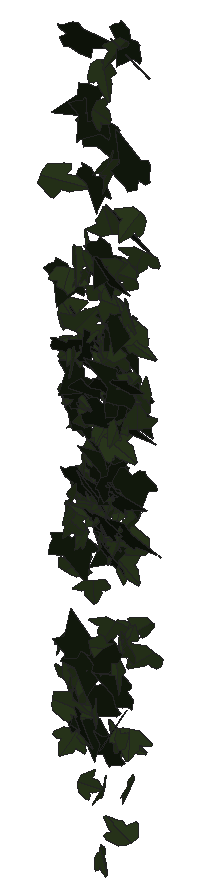
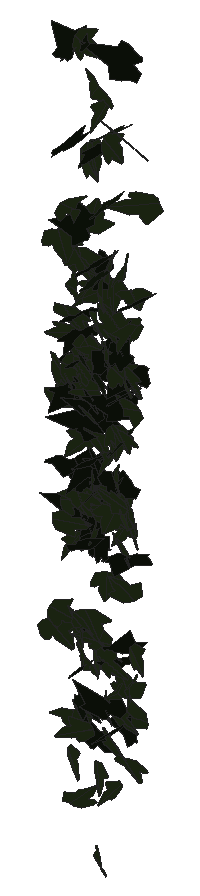
# SketchUp Ruby script. Lengths in inches.
U = 1.inch
M = Sketchup.active_model
def pt(a) = Geom::Point3d.new(a.map { |v| v * U })
def face(e, loops, mat)
  f = e.add_face(loops[0].map { |a| pt(a) })
  loops[1..].each { |l| e.add_face(l.map { |a| pt(a) }).erase! }
  f.material = f.back_material = mat if mat
  f
end
# faces: each face lists its corners as indices into pts; further lists are holes
def faces(e, pts, list, mat = nil) = list.each { |f| face(e, (f[0].is_a?(Array) ? f : [f]).map { |l| l.map { |i| pts[i] } }, mat) }
# xy, xz, yz: faces in a plane at the given z, y or x. An outline is a flat list of corners, or four numbers for a rectangle; further outlines are holes
def ring(l) = l.size == 4 ? [[l[0], l[1]], [l[2], l[1]], [l[2], l[3]], [l[0], l[3]]] : l.each_slice(2).to_a
def flat(e, list, mat, &to3) = list.each { |f| face(e, (f[0].is_a?(Array) ? f : [f]).map { |l| ring(l).map { |u, v| to3.(u, v) } }, mat) }
def xy(e, z, list, mat = nil) = flat(e, list, mat) { |x, y| [x, y, z] }
def xz(e, y, list, mat = nil) = flat(e, list, mat) { |x, z| [x, y, z] }
def yz(e, x, list, mat = nil) = flat(e, list, mat) { |y, z| [x, y, z] }
def lines(e, pts, list) = list.each { |a, b| e.add_line(pt(pts[a]), pt(pts[b])) }
# prism: a flat outline (further loops are holes) pulled along v
def prism(e, loops, v, mat = nil)
  f = face(e, loops, mat); d = Geom::Vector3d.new(v.map { |x| x * U })
  f.pushpull(f.normal.samedirection?(d) ? d.length : -d.length)
end
def box(e, o, s, mat = nil) = prism(e, [[o, [o[0] + s[0], o[1], o[2]], [o[0] + s[0], o[1] + s[1], o[2]], [o[0], o[1] + s[1], o[2]]]], [0, 0, s[2]], mat)
def at(x, y, z, deg = 0) = Geom::Transformation.translation(pt([x, y, z])) * Geom::Transformation.rotation(ORIGIN, Z_AXIS, deg.degrees)
def axes(o, x, y, z) = Geom::Transformation.new([*x, 0, *y, 0, *z, 0, *pt(o).to_a, 1])
def part(name) = M.definitions.add(name)
# library, detail: a bought-in or finely detailed component or shape, given as its bounding box
def library(name, o, s) = part(name).tap { |d| box(d.entities, o, s) }
def detail(e, o, s) = box(e.add_group.entities, o, s)
def put(e, d, t, mat = nil) = e.add_instance(d, t).tap { |i| i.material = mat if mat }
def group(e, t, mat = nil) = e.add_group.tap { |g| g.transformation = t; g.material = mat if mat }.entities
root = M.entities
M.materials.add("1026 AP 7946 SUNNY SIDE UP").color = [254, 231, 186]
M.materials.add("efeu1").color = [18, 25, 13]
M.materials.add("efeu2").color = [43, 57, 29]
c1 = part("ivyleaf_10")
p = [[0,0.5,-0.03],[-0.0625,2.02,-0.43],[-0.19,2.01,-0.46],[-0.54,1.05,-0.29],[-0.52,0.625,-0.18],[-0.83,0.76,-0.28],
  [-1.16,0.64,-0.33],[-1.15,0.33,-0.24],[-0.77,-0.39,0.02],[-0.3,-0.51,0.16],[0.04,-0.48,0.23],[-0.02,2.01,-0.4375],
  [-0.06,2.01,-0.43],[0.04,-0.49,0.23],[0.67,-0.49,0.14],[1.38,0.36,-0.2],[1.375,0.51,-0.24],[0.81,0.65,-0.19],
  [0.62,0.59,-0.15],[0.6,1.09,-0.28],[0.5,1.23,-0.31]]
faces(c1.entities,p,[[0,1,2,3,4,5,6,7,8,9,10],[11,12,0,13,14,15,16,17,18,19,20]],"efeu2")
c2 = part("ivyleaf_9")
p = [[1.54,2.16,1.25],[1.36,2.04,1.19],[-0.21,0.99,0.68],[-0.71,1.11,0.82],[-0.85,0.86,0.67],[-0.8,0.17,0.21],
  [-0.9,-0.01,0.1],[-0.67,-0.16,-0.02],[-0.08,-0.08,-0.05],[-0.03,-0.6,-0.4],[0.65,-0.88,-0.66],[0.83,-0.6,-0.49],
  [1.29,-0.42,-0.43],[1.8125,-0.07,-0.26],[1.21,0.44,0.15]]
faces(c2.entities,p,[[0,1,2,3,4,5,6,7,8,9,10,11,12,13,14]],"efeu1")
put(root,c1,axes([109.62,211.6875,250.39],[0.16374,0.16679,0.12106],[-0.11164,-0.09293,0.20178],[0.29985,-0.12568,0.00902]),"1026 AP 7946 SUNNY SIDE UP")
put(root,c1,axes([108.4,211.74,262.72],[-0.02673,0.24163,-0.15836],[0.017,-0.15471,-0.25045],[-0.45115,-0.02015,-0.00005]),"1026 AP 7946 SUNNY SIDE UP")
put(root,c1,axes([109.34,211.75,256.78],[0.22873,-0.17421,0.08508],[0.06387,-0.07471,-0.23369],[0.29704,0.15022,-0.01527]),"1026 AP 7946 SUNNY SIDE UP")
put(root,c1,axes([108.19,211.72,262.21],[0.27131,0.14604,-0.06363],[-0.05264,-0.05692,-0.2322],[-0.24423,0.1745,-0.02064]),"1026 AP 7946 SUNNY SIDE UP")
put(root,c2,axes([108.61,211.79,257.76],[0.18016,-0.19995,0.08422],[0.04769,-0.07802,-0.23756],[0.33698,0.11794,-0.01141]),"1026 AP 7946 SUNNY SIDE UP")
put(root,c2,axes([108.22,211.78,252.6],[0.01435,-0.02257,-0.25967],[0.39632,-0.02035,0.01116],[-0.03338,-0.25127,0.02093]),"1026 AP 7946 SUNNY SIDE UP")
put(root,c1,axes([108.43,211.59,256.9],[-0.07924,-0.16549,-0.16152],[0.11826,0.1385,-0.17576],[0.33731,-0.08744,0.02368]),"1026 AP 7946 SUNNY SIDE UP")
put(root,c1,axes([109.19,211.67,265.08],[0.00366,-0.24784,-0.05925],[-0.00514,0.05607,-0.25499],[0.39953,0.00299,-0.00274]),"1026 AP 7946 SUNNY SIDE UP")
put(root,c1,axes([109.53,211.81,261.86],[0.08841,-0.06805,0.22834],[0.297,-0.11951,-0.0877],[0.21244,0.19539,0.02759]),"1026 AP 7946 SUNNY SIDE UP")
put(root,c1,axes([108.54,211.67,261.21],[-0.30265,-0.17856,0.11997],[0.11357,0.09444,0.27036],[-0.3163,0.20476,-0.01772]),"1026 AP 7946 SUNNY SIDE UP")
put(root,c2,axes([109.25,211.76,256.22],[0.21365,-0.1787,0.10515],[-0.07433,0.09318,0.23115],[-0.31576,-0.14285,0.01674]),"1026 AP 7946 SUNNY SIDE UP")
put(root,c2,axes([109.39,211.76,256.98],[0.22623,-0.10183,0.19765],[0.23969,-0.11757,-0.18219],[0.24443,0.20954,-0.00427]),"1026 AP 7946 SUNNY SIDE UP")
put(root,c1,axes([108.05,211.68,252.77],[0.01944,0.0241,0.24923],[0.36524,0.06991,-0.019],[-0.11218,0.23179,-0.01869]),"1026 AP 7946 SUNNY SIDE UP")
put(root,c2,axes([109.15,211.77,257.65],[0.1143,-0.06217,0.22835],[0.2682,-0.14212,-0.09936],[0.2439,0.18541,0.00225]),"1026 AP 7946 SUNNY SIDE UP")
put(root,c2,axes([108.92,211.65,257.16],[0.40597,-0.0286,-0.07113],[-0.11167,-0.01843,-0.26645],[0.03583,0.26658,-0.02447]),"1026 AP 7946 SUNNY SIDE UP")
put(root,c2,axes([109.58,211.83,260.13],[-0.13347,-0.27317,-0.03518],[-0.02589,-0.02901,0.29443],[-0.43181,0.08617,-0.00678]),"1026 AP 7946 SUNNY SIDE UP")
put(root,c1,axes([108.83,211.71,255.64],[-0.22701,-0.16897,-0.01737],[0.03319,0.00284,-0.22848],[0.26479,-0.14522,0.01374]),"1026 AP 7946 SUNNY SIDE UP")
put(root,c1,axes([109.25,211.82,264.9375],[0.07697,-0.27103,0.09657],[0.03725,-0.09252,-0.2842],[0.4502,0.05399,0.007]),"1026 AP 7946 SUNNY SIDE UP")
put(root,c2,axes([108.625,211.84,253.9],[-0.16438,-0.22602,-0.02982],[0.03648,0.01971,-0.2561],[0.35618,-0.10633,0.01247]),"1026 AP 7946 SUNNY SIDE UP")
put(root,c2,axes([108.33,211.78,257.66],[0.12623,-0.04783,0.24696],[0.29425,-0.15076,-0.09632],[0.24796,0.20326,-0.01142]),"1026 AP 7946 SUNNY SIDE UP")
put(root,c2,axes([109.29,211.62,260.24],[0.32636,0.14489,-0.05329],[-0.05073,-0.04535,-0.26035],[-0.23698,0.20925,-0.01766]),"1026 AP 7946 SUNNY SIDE UP")
put(root,c2,axes([108.0625,211.91,262.08],[-0.12606,-0.22075,0.10012],[-0.02119,-0.09947,-0.24168],[0.37946,-0.07889,0.01977]),"1026 AP 7946 SUNNY SIDE UP")
put(root,c1,axes([108.14,211.78,259.65],[-0.16249,0.00322,-0.21366],[0.2904,-0.10409,-0.09707],[-0.14854,-0.20704,0.04396]),"1026 AP 7946 SUNNY SIDE UP")
put(root,c1,axes([108.24,211.75,253.33],[-0.30544,-0.02384,0.1197],[0.18237,0.00979,0.20164],[-0.04008,0.22621,0.00523]),"1026 AP 7946 SUNNY SIDE UP")
put(root,c2,axes([108.52,211.6875,254.12],[-0.27032,-0.12765,0.11551],[0.14375,0.06617,0.22097],[-0.22607,0.19471,0.00239]),"1026 AP 7946 SUNNY SIDE UP")
put(root,c1,axes([108.29,211.7,257.0625],[0.17219,-0.1863,-0.09583],[-0.07606,0.07824,-0.22216],[0.31771,0.1197,-0.00125]),"1026 AP 7946 SUNNY SIDE UP")
put(root,c2,axes([109.41,211.82,252.84],[-0.1908,0.11557,-0.18423],[0.18209,-0.13781,-0.17287],[-0.28199,-0.16718,0.01303]),"1026 AP 7946 SUNNY SIDE UP")
put(root,c2,axes([109.27,211.63,254.12],[-0.13737,0.14339,0.17972],[-0.19285,0.1259,-0.16994],[-0.29697,-0.14809,0.02722]),"1026 AP 7946 SUNNY SIDE UP")
put(root,c1,axes([109.08,211.66,251.29],[0.03072,-0.20439,-0.13522],[-0.03077,0.12876,-0.21067],[0.37972,0.02697,-0.00613]),"1026 AP 7946 SUNNY SIDE UP")
put(root,c1,axes([108.08,211.8,254.25],[0.05919,-0.22176,0.04165],[0.00514,-0.04172,-0.23194],[0.35476,0.0376,-0.00359]),"1026 AP 7946 SUNNY SIDE UP")
put(root,c1,axes([109.29,211.64,257.74],[0.10448,-0.14943,-0.1821],[-0.07442,0.17034,-0.16649],[0.35522,0.07964,0.01868]),"1026 AP 7946 SUNNY SIDE UP")
put(root,c1,axes([109.13,211.89,257.33],[-0.01417,-0.14259,0.17478],[-0.02048,-0.16998,-0.14817],[0.34885,-0.01577,-0.0016]),"1026 AP 7946 SUNNY SIDE UP")
put(root,c1,axes([107.85,211.63,264.27],[-0.07843,-0.0737,-0.29054],[0.40455,0.12249,-0.07925],[0.21411,-0.25843,0.04332]),"1026 AP 7946 SUNNY SIDE UP")
put(root,c1,axes([108.875,211.85,257.125],[-0.07152,-0.04279,-0.22505],[-0.32296,-0.07726,0.05926],[-0.13397,0.20908,-0.02272]),"1026 AP 7946 SUNNY SIDE UP")
put(root,c1,axes([109.21,211.72,260.85],[0.3302,-0.106,0.03569],[-0.02774,0.04264,0.24064],[-0.17345,-0.20862,0.02946]),"1026 AP 7946 SUNNY SIDE UP")
put(root,c2,axes([108.74,211.84,262.53],[0.18189,-0.01795,-0.2499],[0.38208,0.0177,0.11818],[0.01305,-0.26807,0.02295]),"1026 AP 7946 SUNNY SIDE UP")
put(root,c2,axes([108.23,211.81,256.35],[-0.10259,-0.21467,-0.12797],[0.0742,0.11408,-0.23022],[0.3819,-0.07984,0.01035]),"1026 AP 7946 SUNNY SIDE UP")
put(root,c2,axes([108.34,211.98,259.9],[-0.16788,-0.14801,0.17285],[-0.08094,-0.16561,-0.18429],[0.34339,-0.11139,0.04107]),"1026 AP 7946 SUNNY SIDE UP")
put(root,c1,axes([109.31,211.92,267.53],[-0.02574,-0.20105,0.16777],[0.00748,-0.16452,-0.20827],[0.4079,-0.00967,0.01441]),"1026 AP 7946 SUNNY SIDE UP")
put(root,c1,axes([108.45,211.8125,256.6],[0.24334,-0.17909,-0.02234],[-0.03947,0.00557,-0.2433],[0.28071,0.15603,-0.01484]),"1026 AP 7946 SUNNY SIDE UP")
put(root,c2,axes([109.44,211.92,253.41],[0.00219,-0.2425,-0.04635],[0.01362,-0.04354,0.24943],[-0.38719,-0.0029,0.00851]),"1026 AP 7946 SUNNY SIDE UP")
put(root,c2,axes([109,211.8125,251.94],[-0.17472,0.07094,0.2166],[0.20905,-0.16644,0.12951],[0.27861,0.16936,0.03866]),"1026 AP 7946 SUNNY SIDE UP")
put(root,c1,axes([109.14,211.86,263.47],[-0.27817,-0.17286,-0.08077],[-0.10981,-0.03895,0.25375],[-0.27684,0.18914,-0.01948]),"1026 AP 7946 SUNNY SIDE UP")
put(root,c1,axes([109.17,211.65,261.99],[0.03389,-0.16642,-0.21659],[0.17901,0.1957,-0.14709],[0.38044,-0.07726,0.0885]),"1026 AP 7946 SUNNY SIDE UP")
put(root,c1,axes([109.57,211.98,260.23],[-0.03599,-0.15707,0.22319],[0.01897,-0.21871,-0.16265],[0.42147,-0.00357,0.02638]),"1026 AP 7946 SUNNY SIDE UP")
put(root,c1,axes([109.43,211.71,252.33],[0.21588,-0.04806,0.18036],[-0.24157,0.08685,0.14895],[-0.15289,-0.20507,0.01934]),"1026 AP 7946 SUNNY SIDE UP")
put(root,c1,axes([108.6,211.85,257.6],[-0.11718,-0.00608,0.25692],[0.38788,-0.04077,0.07467],[0.05875,0.2571,0.01946]),"1026 AP 7946 SUNNY SIDE UP")
put(root,c1,axes([108.23,211.92,257.4375],[0.09795,-0.21074,0.13687],[0.06227,-0.12808,-0.22713],[0.38776,0.0738,0.00191]),"1026 AP 7946 SUNNY SIDE UP")
put(root,c2,axes([109.84,211.77,264.88],[-0.20483,-0.21978,0.15228],[0.09645,0.13664,0.26357],[-0.40628,0.14325,-0.0142]),"1026 AP 7946 SUNNY SIDE UP")
put(root,c1,axes([108.14,211.96,260.35],[0.10367,-0.10719,0.21061],[0.17755,-0.17119,-0.13059],[0.31755,0.13071,0.00426]),"1026 AP 7946 SUNNY SIDE UP")
put(root,c2,axes([109.45,211.97,267.32],[0.03804,-0.16475,0.22395],[0.19609,-0.18842,-0.16182],[0.38276,0.1129,0.06064]),"1026 AP 7946 SUNNY SIDE UP")
put(root,c1,axes([108.85,211.98,253.75],[0.01117,-0.04884,-0.23874],[0.05432,-0.22888,0.0495],[-0.36799,-0.03527,0.00006]),"1026 AP 7946 SUNNY SIDE UP")
put(root,c1,axes([108.26,211.63,253.38],[0.01241,0.07556,-0.23894],[-0.00643,0.2325,0.0791],[0.38415,0.00145,0.00904]),"1026 AP 7946 SUNNY SIDE UP")
put(root,c1,axes([109.61,211.84,251.48],[0.09923,-0.2281,-0.01332],[-0.00865,0.01055,-0.24374],[0.35903,0.0633,-0.00219]),"1026 AP 7946 SUNNY SIDE UP")
put(root,c2,axes([108.62,212.04,265.6875],[-0.1835,-0.18439,0.15708],[-0.02231,-0.16512,-0.21638],[0.37662,-0.09962,0.06372]),"1026 AP 7946 SUNNY SIDE UP")
put(root,c2,axes([108.4,211.68,259.57],[0.05862,0.04047,0.25907],[0.36203,0.10281,-0.05165],[-0.17046,0.23226,-0.02061]),"1026 AP 7946 SUNNY SIDE UP")
put(root,c1,axes([109.58,212.01,257.24],[0.02105,-0.08409,0.22587],[0.04287,-0.21805,-0.08895],[0.36744,0.03026,-0.00256]),"1026 AP 7946 SUNNY SIDE UP")
put(root,c1,axes([108.34,211.9,257.22],[-0.18109,0.05527,0.23907],[0.3584,-0.04938,0.12853],[0.10907,0.25403,-0.02541]),"1026 AP 7946 SUNNY SIDE UP")
put(root,c1,axes([109.57,211.72,256.3],[-0.00172,0.21365,0.13356],[-0.00151,0.12843,-0.21935],[-0.39197,-0.00143,0.00026]),"1026 AP 7946 SUNNY SIDE UP")
put(root,c1,axes([109.59,212.03,263.79],[-0.17414,-0.12477,0.21325],[0.06226,-0.23462,-0.12482],[0.37588,-0.01894,0.11947]),"1026 AP 7946 SUNNY SIDE UP")
put(root,c1,axes([108.89,211.83,262.08],[-0.27123,-0.03838,-0.15814],[0.24628,-0.01147,-0.17869],[0.03292,-0.23048,0.03384]),"1026 AP 7946 SUNNY SIDE UP")
put(root,c1,axes([109.38,211.89,262.73],[-0.30788,-0.09847,0.09167],[-0.10468,-0.06546,-0.22452],[0.18122,-0.20511,0.02605]),"1026 AP 7946 SUNNY SIDE UP")
put(root,c1,axes([109.27,211.83,260.76],[-0.31275,0.01162,0.14131],[-0.21633,-0.01248,-0.20459],[-0.00388,-0.24125,0.01597]),"1026 AP 7946 SUNNY SIDE UP")
put(root,c1,axes([108.88,211.77,254.22],[-0.05608,-0.0056,0.21612],[0.25203,0.13668,0.03262],[-0.21309,0.16313,-0.01829]),"1026 AP 7946 SUNNY SIDE UP")
put(root,c1,axes([108.9375,211.69,266.05],[-0.02164,0.17227,0.19565],[-0.08206,0.18334,-0.17506],[-0.39358,-0.0477,0.02574]),"1026 AP 7946 SUNNY SIDE UP")
put(root,c2,axes([108.53,211.99,252.41],[-0.01757,-0.25082,0.03486],[0.0006,-0.03531,-0.25885],[0.39826,-0.01101,0.00193]),"1026 AP 7946 SUNNY SIDE UP")
put(root,c1,axes([109.01,211.89,257.29],[-0.27358,-0.04492,-0.15363],[-0.23723,-0.00533,0.18328],[-0.0592,0.22892,-0.02448]),"1026 AP 7946 SUNNY SIDE UP")
put(root,c1,axes([109.01,211.74,256.84],[0.06762,-0.16223,-0.17305],[0.05527,0.17246,-0.16221],[0.36197,0.00398,0.05709]),"1026 AP 7946 SUNNY SIDE UP")
put(root,c1,axes([109.64,211.83,262.6],[-0.07969,0.03933,0.23922],[-0.36971,0.00057,-0.05301],[-0.01409,-0.23746,0.03807]),"1026 AP 7946 SUNNY SIDE UP")
put(root,c1,axes([109.74,211.91,259.38],[-0.25423,-0.16936,-0.02964],[-0.04206,-0.01288,0.2409],[-0.26658,0.16355,-0.00973]),"1026 AP 7946 SUNNY SIDE UP")
put(root,c1,axes([109.24,211.9375,259.31],[0.36203,-0.14746,0.04088],[0.03321,-0.04187,-0.28086],[0.23815,0.23,-0.02298]),"1026 AP 7946 SUNNY SIDE UP")
put(root,c1,axes([108.96,211.9375,261.46],[0.19435,-0.19145,0.05007],[0.02964,-0.04692,-0.23484],[0.30959,0.12468,-0.00895]),"1026 AP 7946 SUNNY SIDE UP")
put(root,c2,axes([109.23,211.99,258.1],[-0.10213,-0.25219,-0.03682],[-0.02354,-0.03156,0.26801],[-0.3995,0.06633,-0.00638]),"1026 AP 7946 SUNNY SIDE UP")
put(root,c1,axes([108.41,211.89,257.61],[-0.19582,0.00845,-0.20896],[0.30531,-0.06471,-0.12594],[-0.09345,-0.22909,0.02642]),"1026 AP 7946 SUNNY SIDE UP")
put(root,c1,axes([109.14,211.96,253.83],[0.26663,-0.09,0.14469],[0.18596,-0.07742,-0.19793],[0.18595,0.20647,-0.00954]),"1026 AP 7946 SUNNY SIDE UP")
put(root,c1,axes([108.35,212.02,258.1],[0.09552,-0.12232,0.19498],[0.18733,-0.14979,-0.13949],[0.30186,0.13167,0.02487]),"1026 AP 7946 SUNNY SIDE UP")
put(root,c2,axes([109.29,212.04,261.49],[-0.14549,-0.22997,0.04724],[-0.00721,-0.04891,-0.25527],[0.36907,-0.09161,0.01363]),"1026 AP 7946 SUNNY SIDE UP")
put(root,c1,axes([108.52,211.7,253.16],[0.02559,0.03935,-0.22653],[0.07022,0.21568,0.04438],[0.34451,-0.04688,0.00778]),"1026 AP 7946 SUNNY SIDE UP")
put(root,c2,axes([109.24,211.97,259.82],[-0.22884,-0.00426,-0.20785],[0.31634,-0.02211,-0.14917],[-0.0243,-0.24776,0.01543]),"1026 AP 7946 SUNNY SIDE UP")
put(root,c1,axes([109.58,211.79,254.5],[-0.2336,0.11119,0.17761],[-0.25029,0.07058,-0.18848],[-0.20217,-0.21586,0.02812]),"1026 AP 7946 SUNNY SIDE UP")
put(root,c2,axes([109.22,211.7,258.15],[0.03638,-0.04572,-0.29356],[-0.20068,0.25449,-0.0513],[0.40657,0.1297,0.00095]),"1026 AP 7946 SUNNY SIDE UP")
put(root,c1,axes([109.15,211.91,254.76],[-0.30074,-0.09288,0.08544],[-0.10248,-0.05597,-0.21836],[0.16748,-0.20103,0.0198]),"1026 AP 7946 SUNNY SIDE UP")
put(root,c1,axes([108.56,212.03,252.92],[0.11903,-0.08271,0.22439],[0.25192,-0.14848,-0.11607],[0.26694,0.17701,0.00948]),"1026 AP 7946 SUNNY SIDE UP")
put(root,c1,axes([108.53,211.81,260.95],[0.28741,-0.0914,0.11703],[-0.12996,0.08611,0.20793],[-0.18964,-0.19753,0.03487]),"1026 AP 7946 SUNNY SIDE UP")
put(root,c2,axes([108.13,211.84,267.39],[0.26914,0.04743,-0.21351],[0.25799,0.14026,0.17326],[0.21326,-0.22954,0.05985]),"1026 AP 7946 SUNNY SIDE UP")
put(root,c2,axes([108.6,212,260.54],[0.12312,0.12267,0.24795],[-0.24023,-0.18567,0.14804],[0.34913,-0.17102,0.01443]),"1026 AP 7946 SUNNY SIDE UP")
put(root,c1,axes([108.14,211.77,261.41],[0.05154,0.25749,0.12255],[0.00558,0.11789,-0.2665],[-0.445,0.0313,0.01085]),"1026 AP 7946 SUNNY SIDE UP")
put(root,c2,axes([108.94,212.11,262.7],[-0.14117,-0.23407,0.13978],[-0.06277,-0.13135,-0.25888],[0.42182,-0.09788,0.00826]),"1026 AP 7946 SUNNY SIDE UP")
put(root,c1,axes([109.51,211.92,252.48],[0.30954,0.11816,0.00205],[0.01765,-0.01614,-0.23576],[-0.18496,0.1962,-0.01906]),"1026 AP 7946 SUNNY SIDE UP")
put(root,c1,axes([109.73,211.99,256.71],[0.00368,0.02792,0.24173],[-0.28655,-0.14891,0.01927],[0.23613,-0.18114,0.01962]),"1026 AP 7946 SUNNY SIDE UP")
put(root,c2,axes([108.13,211.8,260.64],[0.37454,0.11133,-0.02881],[-0.02572,-0.03231,-0.27009],[-0.1789,0.23772,-0.02149]),"1026 AP 7946 SUNNY SIDE UP")
put(root,c2,axes([109.55,211.98,258.13],[-0.17674,-0.19929,-0.1048],[0.10934,0.07577,-0.23424],[0.33356,-0.13044,0.02125]),"1026 AP 7946 SUNNY SIDE UP")
put(root,c2,axes([108.7,212.06,256.38],[-0.07928,0.02725,0.27831],[0.04197,-0.27279,0.0319],[0.42463,0.03205,0.04881]),"1026 AP 7946 SUNNY SIDE UP")
put(root,c1,axes([108.46,211.86,252.8125],[0.11981,-0.0725,-0.20186],[-0.26321,0.1029,-0.1059],[0.19557,0.1829,-0.01886]),"1026 AP 7946 SUNNY SIDE UP")
put(root,c2,axes([108.64,211.81,259.32],[0.26046,0.09753,-0.17691],[0.13398,0.16764,0.18315],[0.28098,-0.17034,0.07666]),"1026 AP 7946 SUNNY SIDE UP")
put(root,c1,axes([108.5,211.88,262.33],[-0.0123,-0.24365,-0.0843],[0.03295,0.07961,-0.25002],[0.40211,-0.01398,0.01791]),"1026 AP 7946 SUNNY SIDE UP")
put(root,c1,axes([109.59,211.96,261.4375],[0.37608,-0.05168,-0.08033],[-0.12683,-0.00706,-0.25102],[0.07375,0.25138,-0.02203]),"1026 AP 7946 SUNNY SIDE UP")
put(root,c1,axes([108.71,211.81,262.6],[-0.12635,0.24935,-0.12174],[-0.05338,0.1147,0.27055],[0.43156,0.08719,-0.00218]),"1026 AP 7946 SUNNY SIDE UP")
put(root,c1,axes([108.63,211.8,258.48],[-0.03919,0.15722,0.15847],[-0.03992,0.15082,-0.1631],[-0.34256,-0.03556,0.00088]),"1026 AP 7946 SUNNY SIDE UP")
put(root,c1,axes([108.45,211.93,259.08],[-0.09189,-0.23966,-0.03925],[0.01213,0.03594,-0.25392],[0.38105,-0.05894,-0.00138]),"1026 AP 7946 SUNNY SIDE UP")
put(root,c2,axes([108.77,212.11,262.46],[0.02359,-0.22745,0.12634],[0.04679,-0.1218,-0.23472],[0.40459,0.02735,0.01978]),"1026 AP 7946 SUNNY SIDE UP")
put(root,c1,axes([108.21,211.93,260.52],[0.25936,-0.10675,-0.12725],[-0.16571,0.06336,-0.20201],[0.19512,0.19571,-0.00241]),"1026 AP 7946 SUNNY SIDE UP")
put(root,c2,axes([109.21,212.11,256.44],[-0.26485,-0.14127,0.10708],[-0.10019,-0.08615,-0.22578],[0.25774,-0.17866,0.02226]),"1026 AP 7946 SUNNY SIDE UP")
put(root,c1,axes([109.39,212.01,254.74],[0.32554,-0.09518,0.05858],[0.06878,-0.0418,-0.23416],[0.16067,0.21074,-0.01845]),"1026 AP 7946 SUNNY SIDE UP")
put(root,c2,axes([108.52,212.02,257.92],[-0.03119,0.0951,0.2511],[0.13315,-0.22839,0.09778],[0.38843,0.08592,-0.01336]),"1026 AP 7946 SUNNY SIDE UP")
put(root,c1,axes([108.08,211.98,251.92],[0.33482,-0.04921,-0.04259],[-0.07034,-0.01208,-0.22413],[0.07218,0.21652,-0.02085]),"1026 AP 7946 SUNNY SIDE UP")
put(root,c1,axes([108.27,212.08,260.57],[-0.12832,-0.17522,0.15631],[-0.00935,-0.16024,-0.1936],[0.36536,-0.06564,0.04994]),"1026 AP 7946 SUNNY SIDE UP")
put(root,c1,axes([108.76,211.99,260.79],[0.36195,0.09555,0.03932],[0.06916,-0.00828,-0.25559],[-0.14591,0.2331,-0.0236]),"1026 AP 7946 SUNNY SIDE UP")
put(root,c1,axes([109.08,212.05,260.21],[-0.13495,0.02517,0.22292],[0.32047,-0.07243,0.09159],[0.12034,0.22109,0.00608]),"1026 AP 7946 SUNNY SIDE UP")
put(root,c1,axes([109.93,212.02,254.34],[-0.26293,-0.0768,0.15555],[-0.19822,-0.08622,-0.18896],[0.17884,-0.20847,0.01925]),"1026 AP 7946 SUNNY SIDE UP")
put(root,c1,axes([108.68,212.09,249.48],[0.09447,-0.01664,0.22556],[0.27292,-0.1356,-0.06045],[0.21172,0.18222,-0.02272]),"1026 AP 7946 SUNNY SIDE UP")
put(root,c1,axes([108.47,212.1,265.59],[0.00488,-0.22114,0.14215],[0.02389,-0.13886,-0.22836],[0.41021,0.01072,0.01161]),"1026 AP 7946 SUNNY SIDE UP")
put(root,c1,axes([108.51,211.82,251.11],[-0.01312,0.11415,0.19682],[-0.00871,0.19037,-0.11671],[-0.34896,-0.00904,-0.00449]),"1026 AP 7946 SUNNY SIDE UP")
put(root,c1,axes([108.5,212.1,260.77],[0.0965,-0.04044,0.22357],[0.28976,-0.11506,-0.07637],[0.19175,0.19422,0.00289]),"1026 AP 7946 SUNNY SIDE UP")
put(root,c1,axes([110,211.86,260.04],[-0.01901,0.0501,0.27544],[-0.38254,0.11711,-0.03329],[-0.19035,-0.24034,0.03939]),"1026 AP 7946 SUNNY SIDE UP")
put(root,c2,axes([108.95,212.2,257.55],[-0.08854,-0.12743,0.22261],[-0.07361,-0.21299,-0.14273],[0.38853,-0.06939,0.02369]),"1026 AP 7946 SUNNY SIDE UP")
put(root,c2,axes([108.17,212.02,259.0625],[0.20129,-0.23089,-0.06436],[-0.05853,0.04926,-0.27155],[0.37099,0.13305,-0.00792]),"1026 AP 7946 SUNNY SIDE UP")
put(root,c2,axes([108.31,212.09,260.81],[0.28158,-0.20851,0.06181],[-0.02663,0.06565,0.28193],[-0.34064,-0.17748,0.02906]),"1026 AP 7946 SUNNY SIDE UP")
put(root,c1,axes([108.75,211.91,253.95],[0.06574,-0.04326,-0.25856],[-0.32554,0.14193,-0.05996],[0.23257,0.21088,-0.01084]),"1026 AP 7946 SUNNY SIDE UP")
put(root,c1,axes([108.7,212.1,266.75],[0.31489,-0.08048,0.1965],[0.26563,-0.09097,-0.22226],[0.18932,0.26151,-0.01499]),"1026 AP 7946 SUNNY SIDE UP")
put(root,c1,axes([108.08,211.95,255.62],[-0.19155,-0.11744,0.12782],[0.12786,0.0951,0.17459],[-0.23713,0.14614,-0.00912]),"1026 AP 7946 SUNNY SIDE UP")
put(root,c1,axes([109.78,212.02,263.05],[-0.34537,-0.06147,0.0713],[-0.09431,-0.0424,-0.23395],[0.11141,-0.22646,0.02299]),"1026 AP 7946 SUNNY SIDE UP")
put(root,c1,axes([109.07,211.91,259.83],[0.05233,0.0046,0.22702],[0.25362,0.15135,-0.02747],[-0.23615,0.16356,0.02081]),"1026 AP 7946 SUNNY SIDE UP")
put(root,c1,axes([108.3,212.02,252.06],[0.28686,-0.14098,-0.07842],[0.1219,-0.02191,0.23556],[-0.2198,-0.19615,0.0283]),"1026 AP 7946 SUNNY SIDE UP")
put(root,c2,axes([108.48,212.19,264.21],[-0.01253,-0.22977,0.11436],[0.01246,-0.11254,-0.23726],[0.40196,-0.00368,0.01092]),"1026 AP 7946 SUNNY SIDE UP")
put(root,c1,axes([108.22,212.07,257.63],[0.07284,-0.04896,-0.22075],[0.30963,-0.08742,0.06401],[-0.1526,-0.20075,0.0245]),"1026 AP 7946 SUNNY SIDE UP")
put(root,c2,axes([108.59,211.96,252.83],[-0.17849,0.06161,0.24237],[0.35663,-0.06581,0.1303],[0.13652,0.25246,-0.02351]),"1026 AP 7946 SUNNY SIDE UP")
put(root,c2,axes([109.23,212.04,261.12],[0.00318,-0.2188,-0.12758],[-0.01412,0.12246,-0.22459],[0.39411,0.00616,-0.00702]),"1026 AP 7946 SUNNY SIDE UP")
put(root,c1,axes([109.42,212.04,261.05],[-0.17156,-0.05318,-0.19572],[0.30956,-0.03706,-0.10618],[-0.01089,-0.21566,0.06513]),"1026 AP 7946 SUNNY SIDE UP")
put(root,c1,axes([108.42,212.01,257.36],[-0.34189,-0.0539,-0.05561],[0.09005,-0.00901,-0.22972],[0.07872,-0.22378,0.02125]),"1026 AP 7946 SUNNY SIDE UP")
put(root,c1,axes([108.17,212.08,259.24],[0.32847,-0.08471,0.01118],[0.00481,-0.0225,-0.23147],[0.1343,0.20799,-0.01905]),"1026 AP 7946 SUNNY SIDE UP")
put(root,c2,axes([109.05,212.12,263.54],[0.26683,-0.14922,0.14934],[0.14283,-0.11637,-0.23226],[0.29533,0.1911,-0.0226]),"1026 AP 7946 SUNNY SIDE UP")
put(root,c1,axes([109.11,211.89,258.78],[0.10685,0.20317,0.19299],[0.09973,0.17508,-0.21965],[-0.42168,0.09289,-0.00304]),"1026 AP 7946 SUNNY SIDE UP")
put(root,c2,axes([108.88,212.03,259.21],[0.31811,-0.05245,0.16645],[0.22911,-0.07647,-0.21359],[0.13817,0.24756,-0.02906]),"1026 AP 7946 SUNNY SIDE UP")
put(root,c2,axes([109.36,212.01,259.78],[-0.05151,-0.18027,-0.20691],[0.08861,0.19224,-0.18705],[0.41378,-0.06361,0.0143]),"1026 AP 7946 SUNNY SIDE UP")
put(root,c2,axes([108.65,212.04,265.47],[0.06939,-0.22266,-0.1442],[-0.00288,0.14039,-0.23195],[0.41248,0.03844,0.02264]),"1026 AP 7946 SUNNY SIDE UP")
put(root,c1,axes([108.6,212.2,262.23],[0.1026,-0.13421,0.22437],[0.21502,-0.17258,-0.15225],[0.34118,0.14913,0.02848]),"1026 AP 7946 SUNNY SIDE UP")
put(root,c1,axes([109.7,212.19,254.83],[-0.0635,-0.13326,0.19215],[-0.06709,-0.1825,-0.14433],[0.35514,-0.0583,0.0071]),"1026 AP 7946 SUNNY SIDE UP")
put(root,c2,axes([109.1,211.875,260.29],[-0.06906,0.18693,0.18685],[-0.10249,0.16908,-0.19595],[-0.39531,-0.07649,0.01816]),"1026 AP 7946 SUNNY SIDE UP")
put(root,c2,axes([108.56,212.07,265.97],[-0.36639,0.12872,0.0327],[-0.06522,-0.01136,-0.27258],[-0.19772,-0.23479,0.02932]),"1026 AP 7946 SUNNY SIDE UP")
put(root,c1,axes([109.2,212.09,257.51],[0.35481,0.06527,-0.01383],[-0.01203,-0.02304,-0.24125],[-0.10421,0.22489,-0.01926]),"1026 AP 7946 SUNNY SIDE UP")
put(root,c1,axes([108.8,212.09,258.98],[0.35347,-0.02217,-0.03378],[-0.05378,-0.01504,-0.23205],[0.031,0.22666,-0.01736]),"1026 AP 7946 SUNNY SIDE UP")
put(root,c2,axes([109.25,212.28,267.48],[-0.06839,-0.19704,0.18904],[-0.05925,-0.18074,-0.20893],[0.42042,-0.05752,0.00131]),"1026 AP 7946 SUNNY SIDE UP")
put(root,c1,axes([109.2,211.9375,252.22],[0.07833,0.07126,0.21762],[0.19742,0.16939,-0.08855],[-0.28894,0.13506,-0.00151]),"1026 AP 7946 SUNNY SIDE UP")
